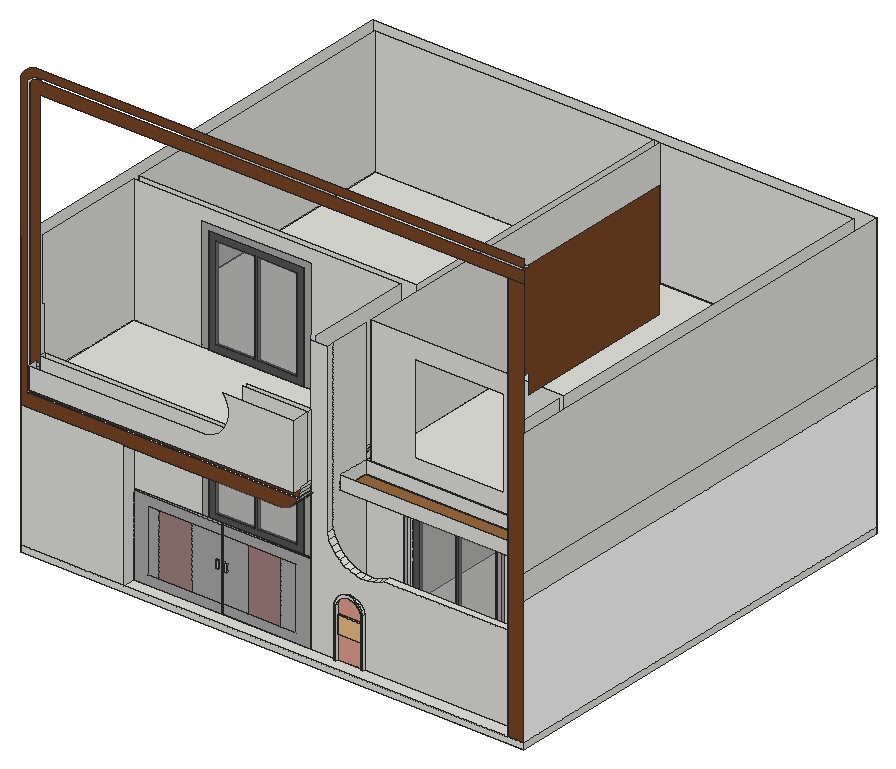
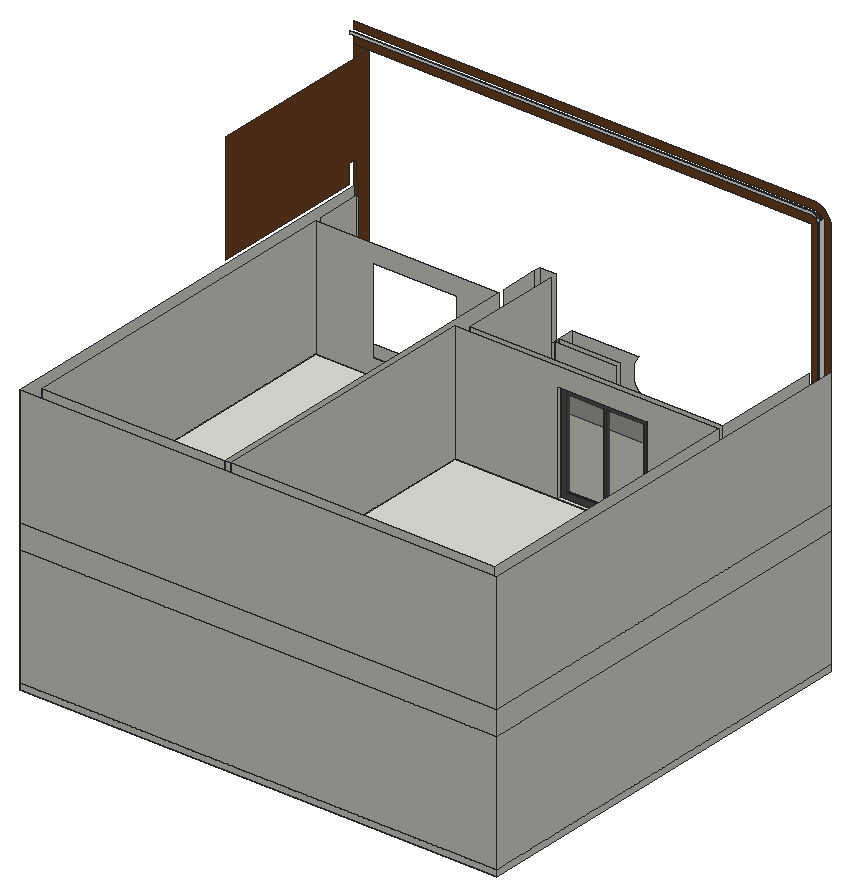
# SketchUp Ruby script. Lengths in millimetres.
U = 1.mm
M = Sketchup.active_model
def pt(a) = Geom::Point3d.new(a.map { |v| v * U })
def face(e, loops, mat)
  f = e.add_face(loops[0].map { |a| pt(a) })
  loops[1..].each { |l| e.add_face(l.map { |a| pt(a) }).erase! }
  f.material = f.back_material = mat if mat
  f
end
# faces: each face lists its corners as indices into pts; further lists are holes
def faces(e, pts, list, mat = nil) = list.each { |f| face(e, (f[0].is_a?(Array) ? f : [f]).map { |l| l.map { |i| pts[i] } }, mat) }
# xy, xz, yz: faces in a plane at the given z, y or x. An outline is a flat list of corners, or four numbers for a rectangle; further outlines are holes
def ring(l) = l.size == 4 ? [[l[0], l[1]], [l[2], l[1]], [l[2], l[3]], [l[0], l[3]]] : l.each_slice(2).to_a
def flat(e, list, mat, &to3) = list.each { |f| face(e, (f[0].is_a?(Array) ? f : [f]).map { |l| ring(l).map { |u, v| to3.(u, v) } }, mat) }
def xy(e, z, list, mat = nil) = flat(e, list, mat) { |x, y| [x, y, z] }
def xz(e, y, list, mat = nil) = flat(e, list, mat) { |x, z| [x, y, z] }
def yz(e, x, list, mat = nil) = flat(e, list, mat) { |y, z| [x, y, z] }
def lines(e, pts, list) = list.each { |a, b| e.add_line(pt(pts[a]), pt(pts[b])) }
# prism: a flat outline (further loops are holes) pulled along v
def prism(e, loops, v, mat = nil)
  f = face(e, loops, mat); d = Geom::Vector3d.new(v.map { |x| x * U })
  f.pushpull(f.normal.samedirection?(d) ? d.length : -d.length)
end
def box(e, o, s, mat = nil) = prism(e, [[o, [o[0] + s[0], o[1], o[2]], [o[0] + s[0], o[1] + s[1], o[2]], [o[0], o[1] + s[1], o[2]]]], [0, 0, s[2]], mat)
def at(x, y, z, deg = 0) = Geom::Transformation.translation(pt([x, y, z])) * Geom::Transformation.rotation(ORIGIN, Z_AXIS, deg.degrees)
def axes(o, x, y, z) = Geom::Transformation.new([*x, 0, *y, 0, *z, 0, *pt(o).to_a, 1])
def part(name) = M.definitions.add(name)
# library, detail: a bought-in or finely detailed component or shape, given as its bounding box
def library(name, o, s) = part(name).tap { |d| box(d.entities, o, s) }
def detail(e, o, s) = box(e.add_group.entities, o, s)
def put(e, d, t, mat = nil) = e.add_instance(d, t).tap { |i| i.material = mat if mat }
def group(e, t, mat = nil) = e.add_group.tap { |g| g.transformation = t; g.material = mat if mat }.entities
root = M.entities
M.materials.add("[0026_LightSalmon]").color = [225, 160, 143]
M.materials.add("[Color M00]").color = [255, 255, 255]
M.materials.add("[Color M03]").color = [170, 170, 170]
M.materials.add("[Color M06]").color = [86, 86, 86]
M.materials.add("[Metal Corrugated Shiny]").color = [193, 193, 193]
M.materials.add("[Translucent Glass Gray]").color = [128, 128, 128]
M.materials["[Translucent Glass Gray]"].alpha = 0.5
M.materials.add("[Wood Floor]").color = [155, 105, 61]
M.materials.add("[Wood Veneer 01]").color = [120, 70, 37]
M.materials.add("[Wood Veneer 02]").color = [163, 128, 128]
c1 = part("Group\#1")
xy(c1.entities,0,[[0,0,1355.7,60.3]],"[Color M06]")
xy(c1.entities,100.1,[[100.1,0,655.5,60.3],[696.9,0,1255.7,60.3]],"[Color M06]")
xy(c1.entities,1517.6,[[100.1,0,655.5,60.3],[696.9,0,1255.7,60.3]],"[Color M06]")
xy(c1.entities,1617.7,[[0,0,1355.7,60.3]],"[Color M06]")
xz(c1.entities,0,[[[0,0,1355.7,1617.7],[696.9,100.1,1255.7,1517.6],[100.1,100.1,655.5,1517.6]]],"[Color M06]")
xz(c1.entities,0,[[100.1,100.1,655.5,1517.6],[696.9,100.1,1255.7,1517.6]],"[Translucent Glass Gray]")
xz(c1.entities,60.3,[[[0,0,1355.7,1617.7],[696.9,100.1,1255.7,1517.6],[100.1,100.1,655.5,1517.6]]],"[Color M06]")
yz(c1.entities,0,[[0,0,60.3,1617.7]],"[Color M06]")
yz(c1.entities,100.1,[[0,100.1,60.3,1517.6]],"[Color M06]")
yz(c1.entities,655.5,[[0,100.1,60.3,1517.6]],"[Color M06]")
yz(c1.entities,696.9,[[0,100.1,60.3,1517.6]],"[Color M06]")
yz(c1.entities,1255.7,[[0,100.1,60.3,1517.6]],"[Color M06]")
yz(c1.entities,1355.7,[[0,0,60.3,1617.7]],"[Color M06]")
c2 = library("61A",[37.8,0,0],[1466.5,605.7,101.6])
xy(root,0,[[3.3,209.6,12195.3,10877.6]])
xy(root,152.4,[[[3.3,209.6,3.3,10877.6,12195.3,10877.6,12195.3,209.6,11814.3,209.6,11814.3,514.4,11890.5,514.4,11890.5,687.4,6787.6,687.4,6787.6,3257.6,4426,3257.6,4426,3410,7047,3410,7047,10572.8,7199.4,10572.8,7199.4,1809.8,11890.5,1809.8,11890.5,10572.8,308.1,10572.8,308.1,3410,2137.7,3410,2137.7,3257.6,308.1,3257.6,308.1,514.4,2505.2,514.4,2505.2,209.6],[7199.4,698.5,11890.5,1657.4]],[2505.2,209.6,11814.3,209.6,11814.3,514.4,8100.8,514.4,8100.8,463.6,8038.4,463.6,8038.4,514.4,7446.1,514.4,7446.1,463.6,7383.6,463.6,7383.6,514.4,2505.2,514.4],[7383.6,463.6,7446.1,514.4],[8038.4,463.6,8100.8,514.4],[308.1,514.4,6787.6,3257.6],
  [6787.6,514.4,11890.5,687.4],[7199.4,698.5,11890.5,1657.4],[7199.4,1809.8,11890.5,10572.8],[2137.7,3257.6,4426,3410],[308.1,3410,7047,10572.8]])
xy(root,543.9,[[8185.1,1603.4,10552.1,1657.4]])
xy(root,759.3,[[8275.8,1657.4,10434.8,1809.8]])
xy(root,759.3,[[8275.8,1603.4,10434.8,1657.4]],"[Color M03]")
xy(root,2234.1,[[8561.3,514.4,11890.5,687.4]])
xy(root,2700.1,[[2137.7,3257.5,4426,3409.9]])
xy(root,3162.7,[[8275.8,1603.4,10434.8,1657.4],[8275.8,1657.4,10434.8,1809.8]])
xy(root,3200.4,[[2505.2,209.6,2505.2,514.4,308.1,514.4,308.1,3257.6,6237.2,3257.6,6237.2,209.6]])
xy(root,3271.3,[[8185.1,1603.4,10552.1,1657.4]],"[Color M03]")
xy(root,3514.6,[[181.8,209.6,6734,325.4]],"[Color M00]")
xy(root,3559,[[241.3,209.6,6734,325.4]],"[Color M00]")
xy(root,3584.1,[[7199.4,887.4,11890.5,1657.4]],"[Wood Floor]")
xy(root,3752.8,[[374.7,0,6787.6,209.6]])
xy(root,3810,[[308.1,424.6,6787.6,555.6],[308.1,555.6,6787.6,555.6,6787.6,3257.6,4426,3257.6,2137.7,3257.5,1971.4,3257.5,308.1,3257.6],[7199.4,1809.8,11890.5,10572.8],[2137.7,3257.5,4426,3257.6,4426,3410,2137.7,3410],[308.1,3410,7047,10572.8]])
xz(root,0,[[374.7,3752.8,6787.6,3752.8,6787.6,5334,5080.9,5334,5145.9,5230.5,5190.6,5116.7,5213.7,4996.7,5214.2,4874.4,5192.2,4754.2,5148.4,4640.1,5084.4,4536,5002.2,4445.4,4904.8,4371.6,4795.5,4317,4677.9,4283.4,4556.2,4272.1,374.7,4272.1]])
xz(root,209.6,[[3.3,0,12195.3,152.4],[3.3,152.4,2505.2,3200.4],[374.7,3752.8,6787.6,3810]])
xz(root,209.6,[[11814.3,152.4,12195.3,10096.5],[3.3,3200.4,6237.2,3200.4,6314.1,3205.8,6389.5,3221.8,6461.9,3248.1,6530,3284.2,6592.3,3329.4,6647.8,3382.9,6695.4,3443.6,6734,3510.2,6763,3581.6,6781.8,3656.4,6790,3733,6787.6,3810,6787.6,3752.8,374.7,3752.8,374.7,4272.1,479.5,4272.1,479.5,10096.5,12195.3,10096.5,12195.3,10388.1,531,10388.1,503.8,10394.3,476.2,10397.6,448.3,10397.9,420.5,10395,393.2,10389.2,366.8,10380.4,341.4,10368.8,317.5,10354.5,295.2,10337.7,275,10318.5,257,10297.2,241.3,10274.1,241.3,3559,6734,3559,6734,3514.6,181.8,3514.6,181.8,10303.9,202.4,10329.9,219.1,10347.4,225.2,10353.9,250.2,10375.7,277.2,10395,305.8,10411.7,335.8,10425.7,367.1,10436.8,399.2,10444.9,431.9,10450,465,10452,498.1,10450.9,531,10446.7,12195.3,10446.7,12195.3,10642.6,432,10642.6,373.3,10634.9,306.3,10615.8,242.9,10587,184.5,10549,132.4,10502.9,87.7,10449.5,51.4,10390.1,24.3,10325.9,7.1,10258.4,3.3,10221.2]],"[Wood Veneer 01]")
xz(root,325.4,[[181.8,3514.6,6734,3514.6,6734,3559,241.3,3559,241.3,10274.1,257,10297.2,275,10318.5,295.2,10337.7,317.5,10354.5,341.4,10368.8,366.8,10380.4,393.2,10389.2,420.5,10395,448.3,10397.9,476.2,10397.6,503.8,10394.3,531,10388.1,12195.3,10388.1,12195.3,10446.7,531,10446.7,498.1,10450.9,465,10452,431.9,10450,399.2,10444.9,367.1,10436.8,335.8,10425.7,305.8,10411.7,277.2,10395,250.2,10375.7,225.2,10353.9,219.1,10347.4,202.4,10329.9,181.8,10303.9]],"[Color M00]")
xz(root,424.6,[[308.1,3810,6787.6,3810,6787.6,5334,5214.2,5334,5214.2,4272.1,308.1,4272.1]])
xz(root,463.6,[[7383.6,152.4,7446.1,152.4,7446.1,1349.5,7467.8,1414.6,7503.5,1473.1,7551.6,1522,7609.4,1558.9,7674.1,1581.8,7742.2,1589.6,7810.4,1581.8,7875,1558.9,7932.8,1522,7980.9,1473.1,8016.7,1414.6,8038.4,1349.5,8038.4,152.4,8100.8,152.4,8100.8,1359.7,8073.6,1441.1,8030.4,1511.7,7972.4,1570.8,7902.6,1615.4,7824.5,1643,7742.2,1652.4,7659.9,1643,7581.9,1615.4,7512,1570.8,7454,1511.7,7410.8,1441.1,7383.6,1359.7]])
xz(root,514.4,[[7383.6,90,8100.8,152.4],[308.1,152.4,2505.2,3200.4],[6787.6,152.4,7383.6,152.4,7383.6,1359.7,7410.8,1441.1,7454,1511.7,7512,1570.8,7581.9,1615.4,7659.9,1643,7742.2,1652.4,7824.5,1643,7902.6,1615.4,7972.4,1570.8,8030.4,1511.7,8073.6,1441.1,8100.8,1359.7,8100.8,152.4,11814.3,152.4,11814.3,2234.1,8561.3,2234.1,8432.1,2170,8294.4,2127,8151.7,2106.2,8007.5,2108.2,7865.3,2132.9,7728.9,2179.6,7601.5,2247.2,7486.3,2334.1,7386.2,2438,7303.8,2556.3,7241,2686.2,7199.4,2824.3,7199.4,6858,6787.6,6858,6787.6,3810,6790,3733,6787.6,3709.8],[7383.6,152.4,7383.6,1359.7,7410.8,1441.1,7454,1511.7,7512,1570.8,7581.9,1615.4,7659.9,1643,7742.2,1652.4,7824.5,1643,7902.6,1615.4,7972.4,1570.8,8030.4,1511.7,8073.6,1441.1,8100.8,1359.7,8100.8,152.4,8038.4,152.4,8038.4,1349.5,8016.7,1414.6,7980.9,1473.1,7932.8,1522,7875,1558.9,7810.4,1581.8,7742.2,1589.6,7674.1,1581.8,7609.4,1558.9,7551.6,1522,7503.5,1473.1,7467.8,1414.6,7446.1,1349.5,7446.1,152.4],[11814.3,152.4,11890.5,2234.1],
  [11814.3,2234.1,11890.5,2824.3],[11814.3,2824.3,11890.5,6858]])
xz(root,514.4,[[7446.1,152.4,8038.4,152.4,8038.4,1349.5,8016.7,1414.6,7980.9,1473.1,7932.8,1522,7875,1558.9,7810.4,1581.8,7742.2,1589.6,7674.1,1581.8,7609.4,1558.9,7551.6,1522,7503.5,1473.1,7467.8,1414.6,7446.1,1349.5]],"[0026_LightSalmon]")
xz(root,555.6,[[308.1,3810,308.1,4272.1,5214.2,4272.1,5214.2,5334,6787.6,5334,6787.6,3810]])
xz(root,887.4,[[7199.4,3584.1,11890.5,3899.4]])
xz(root,1603.4,[[[8185.1,543.9,10552.1,3271.3],[8275.8,759.3,10434.8,3162.7]]],"[Color M03]")
xz(root,1657.4,[[[7199.4,152.4,11890.5,3584.1],[8185.1,543.9,10552.1,3271.3]],[[8185.1,543.9,10552.1,3271.3],[8275.8,759.3,10434.8,3162.7]],[7199.4,3584.1,11890.5,3899.4]])
xz(root,1809.8,[[[7199.4,152.4,11890.5,3200.4],[8275.8,759.3,10434.8,3162.7]],[7199.4,3200.4,11890.5,3810]])
xz(root,3257.6,[[6787.6,3709.8,6787.6,3810,6790,3733]])
xz(root,3410,[[308.1,3200.4,7047,3810],[308.1,3810,308.1,6858,7047,6858,7047,3810,4426,3810,4426,6383.1,2137.7,6383.1,2137.7,3810]])
xz(root,10572.8,[[308.1,152.4,7047,3200.4],[7047,152.4,7199.4,3200.4],[7199.4,152.4,11890.5,3200.4],[308.1,3200.4,7047,3810],[7047,3200.4,7199.4,3810],
  [7199.4,3200.4,11890.5,3810],[308.1,3810,7047,6858],[7047,3810,7199.4,6858],[7199.4,3810,11890.5,6858]])
xz(root,10877.6,[[3.3,0,12195.3,152.4],[3.3,152.4,12195.3,3200.4],[3.3,3200.4,12195.3,3810],[3.3,3810,12195.3,6858]])
yz(root,3.3,[[209.6,0,10877.6,152.4],[209.6,152.4,10877.6,3200.4],[209.6,3200.4,10877.6,3810],[209.6,3810,10877.6,6858]])
yz(root,181.8,[[209.6,3514.6,325.4,10303.9]],"[Color M00]")
yz(root,241.3,[[209.6,3559,325.4,10274.1]],"[Color M00]")
yz(root,308.1,[[514.4,152.4,3257.6,3200.4],[3410,152.4,10572.8,3200.4],[514.4,3200.4,3257.6,3810],[3410,3200.4,10572.8,3810],[424.6,3810,555.6,4272.1],
  [555.6,3810,3257.6,3810,3257.6,6858,514.4,6858,514.4,5372.1,555.6,5372.1],[3410,3810,10572.8,6858]])
yz(root,374.7,[[0,3752.8,209.6,4272.1]])
yz(root,2137.7,[[3257.6,152.4,3410,152.4,3409.9,2700.1,3257.5,2700.1],[3257.5,3810,3410,6383.1]])
yz(root,2505.2,[[209.6,152.4,514.4,3200.4]])
yz(root,4426,[[3257.6,152.4,3257.5,2700.1,3409.9,2700.1,3410,152.4],[3257.6,3810,3257.5,6383.1,3410,6383.1,3410,3810]])
yz(root,6734,[[209.6,3514.6,325.4,3559]],"[Color M00]")
yz(root,6787.6,[[514.4,152.4,687.4,3709.8],[687.4,152.4,3257.6,3709.8],[0,3752.8,209.6,3752.8,209.6,3810,424.6,3810,424.6,5334,0,5334],[424.6,3810,514.4,5334],[514.4,3810,555.6,5334],
  [555.6,3810,687.4,5334],[687.4,3810,3257.6,6858]])
yz(root,7047,[[3410,152.4,10572.8,3200.4],[3410,3200.4,10572.8,3810],[3410,3810,10572.8,6858]])
yz(root,7199.4,[[698.5,152.4,1657.4,152.4,1657.4,3584.1,887.4,3584.1,887.4,3899.4,1657.4,3899.4,1657.4,6858,687.4,6858,687.4,2824.3,698.5,2824.3],[1809.8,152.4,10572.8,3200.4],[514.4,2824.3,687.4,6858],[1809.8,3200.4,10572.8,3810],[887.4,3584.1,1657.4,3899.4],
  [1809.8,3810,10572.8,6858]])
yz(root,7383.6,[[463.6,152.4,514.4,1359.7]])
yz(root,7446.1,[[463.6,152.4,514.4,1349.5]])
yz(root,8038.4,[[463.6,152.4,514.4,1349.5]])
yz(root,8100.8,[[463.6,152.4,514.4,1359.7]])
yz(root,8185.1,[[1603.4,543.9,1657.4,3271.3]],"[Color M03]")
yz(root,8275.8,[[1603.4,759.3,1657.4,3162.7],[1657.4,759.3,1809.8,3162.7]])
yz(root,10434.8,[[1657.4,759.3,1809.8,3162.7]])
yz(root,10434.8,[[1603.4,759.3,1657.4,3162.7]],"[Color M03]")
yz(root,10552.1,[[1603.4,543.9,1657.4,3271.3]],"[Color M03]")
yz(root,11814.3,[[209.6,152.4,209.6,10096.5,4760.9,10096.5,4760.9,7289.8,849.3,7289.8,849.3,7765.4,642.9,7765.4,642.9,8839.2,606.3,8839.2,606.3,7765.4,582.5,7765.4,582.5,7289.8,514.4,7289.8,514.4,152.4]],"[Wood Veneer 01]")
yz(root,11890.5,[[514.4,152.4,687.4,2234.1],[698.5,152.4,698.5,2824.3,514.4,2824.3,514.4,6858,1657.4,6858,1657.4,3899.4,1049.4,3899.4,1049.4,5423.4,946.6,5423.4,946.6,3899.4,887.4,3899.4,887.4,3584.1,1657.4,3584.1,1657.4,152.4],[1809.8,152.4,10572.8,3200.4],[1809.8,3200.4,10572.8,3810],[887.4,3584.1,1657.4,3899.4],
  [1809.8,3810,10572.8,6858]])
yz(root,12195.3,[[209.6,0,10877.6,152.4],[209.6,3200.4,10877.6,3810],[209.6,3810,10877.6,6858]])
yz(root,12195.3,[[209.6,152.4,10877.6,3200.4]],"[Color M00]")
p = [[1988.4,3257.6,152.4],[1988.4,3257.6,3.1],[4575.2,3257.6,3.1],[4575.2,3257.6,152.4],[4426,3257.6,152.4],[4426,3257.6,127],
  [2137.7,3257.5,127],[2137.7,3257.6,152.4],[308.1,3257.6,152.4],[1988.4,3257.5,2849.3],[4575.2,3257.5,2849.3],[6787.6,3257.6,152.4],
  [6787.6,3257.6,3709.8],[6781.8,3257.6,3656.4],[6763,3257.6,3581.6],[6734,3257.6,3510.2],[6695.4,3257.6,3443.6],[6647.8,3257.6,3382.9],
  [6592.3,3257.6,3329.4],[6530,3257.6,3284.2],[6461.9,3257.6,3248.1],[6389.5,3257.6,3221.8],[6314.1,3257.6,3205.8],[6237.2,3257.6,3200.4],
  [308.1,3257.6,3200.4],[2137.7,3257.5,2700.1],[4426,3257.5,2700.1],[7047,3410,152.4],[4426,3410,152.4],[4426,3409.9,2700.1],
  [2137.7,3409.9,2700.1],[2137.7,3410,152.4],[308.1,3410,152.4],[308.1,3410,3200.4],[7047,3410,3200.4],[7446.1,514.4,1349.5],
  [7467.8,514.4,1414.6],[7467.8,463.6,1414.6],[7446.1,463.6,1349.5],[8016.7,514.4,1414.6],[8038.4,514.4,1349.5],[8038.4,463.6,1349.5],
  [8016.7,463.6,1414.6],[7410.8,514.4,1441.1],[7383.6,514.4,1359.7],[7383.6,463.6,1359.7],[7410.8,463.6,1441.1],[8100.8,514.4,1359.7],
  [8073.6,514.4,1441.1],[8073.6,463.6,1441.1],[8100.8,463.6,1359.7],[7503.5,514.4,1473.1],[7503.5,463.6,1473.1],[7980.9,514.4,1473.1],
  [7980.9,463.6,1473.1],[7454,514.4,1511.7],[7454,463.6,1511.7],[8030.4,514.4,1511.7],[8030.4,463.6,1511.7],[7551.6,514.4,1522],
  [7551.6,463.6,1522],[7932.8,514.4,1522],[7932.8,463.6,1522],[7512,514.4,1570.8],[7512,463.6,1570.8],[7972.4,514.4,1570.8],
  [7972.4,463.6,1570.8],[7609.4,514.4,1558.9],[7609.4,463.6,1558.9],[7875,514.4,1558.9],[7875,463.6,1558.9],[7674.1,514.4,1581.8],
  [7674.1,463.6,1581.8],[7810.4,514.4,1581.8],[7810.4,463.6,1581.8],[7581.9,514.4,1615.4],[7581.9,463.6,1615.4],[7902.6,514.4,1615.4],
  [7902.6,463.6,1615.4],[7742.2,514.4,1589.6],[7742.2,463.6,1589.6],[7659.9,514.4,1643],[7659.9,463.6,1643],[7824.5,514.4,1643],
  [7824.5,463.6,1643],[7742.2,514.4,1652.4],[7742.2,463.6,1652.4],[8007.5,514.4,2108.2],[8151.7,514.4,2106.2],[8151.7,687.4,2106.2],
  [8007.5,687.4,2108.2],[8294.4,514.4,2127],[8294.4,687.4,2127],[7865.3,514.4,2132.9],[7865.3,687.4,2132.9],[8432.1,514.4,2170],
  [8432.1,687.4,2170],[7728.9,514.4,2179.6],[7728.9,687.4,2179.6],[8561.3,514.4,2234.1],[8561.3,687.4,2234.1],[7601.5,514.4,2247.2],
  [7601.5,687.4,2247.2],[7486.3,514.4,2334.1],[7486.3,687.4,2334.1],[7386.2,514.4,2438],[7386.2,687.4,2438],[7303.8,514.4,2556.3],
  [7303.8,687.4,2556.3],[7241,514.4,2686.2],[7241,687.4,2686.2],[7199.4,514.4,2824.3],[7199.4,687.4,2824.3],[6314.1,209.6,3205.8],
  [6237.2,209.6,3200.4],[308.1,3257.6,3810],[1971.4,3257.5,3810],[1971.4,3257.5,3643.7],[4592.3,3257.5,3643.7],[4592.3,3257.6,3810],
  [6787.6,3257.6,3810],[6389.5,209.6,3221.8],[6461.9,209.6,3248.1],[6530,209.6,3284.2],[6592.3,209.6,3329.4],[6647.8,209.6,3382.9],
  [6695.4,209.6,3443.6],[6734,209.6,3510.2],[6763,209.6,3581.6],[6781.8,209.6,3656.4],[4426,3257.6,3810],[2137.7,3257.5,3810],
  [6787.6,687.4,3709.8],[6787.6,514.4,3709.8],[6790,514.4,3733],[6790,209.6,3733],[6790,687.4,3733],[6790,3257.6,3733],
  [6787.6,514.4,3810],[6787.6,424.6,3810],[6787.6,209.6,3810],[6787.6,687.4,3810],[6787.6,555.6,3810],[11890.5,1809.8,3810],
  [7199.4,1809.8,3810],[7199.4,1809.8,6858],[11890.5,1809.8,6858],[8275.8,1809.7,4242.9],[10434.8,1809.7,4242.9],[10434.8,1809.7,6401.9],
  [8275.8,1809.7,6401.9],[1971.4,3257.5,6549.4],[4592.3,3257.5,6549.4],[6787.6,3257.6,6858],[308.1,3257.6,6858],[2137.7,3257.5,6383.1],
  [4426,3257.5,6383.1],[308.1,209.6,3810],[308.1,424.6,3810]]
faces(root,p,[[0,1,2,3,4,5,6,7],[5,4,7,6],[8,0,9,10,3,11,12,13,14,15,16,17,18,19,20,21,22,23,24],[27,28,29,30,31,32,33,34],[35,36,37,38],[39,40,41,42],[43,44,45,46],[47,48,49,50],
  [36,51,52,37],[53,39,42,54],[55,43,46,56],[48,57,58,49],[51,59,60,52],[61,53,54,62],[63,55,56,64],[57,65,66,58],
  [59,67,68,60],[69,61,62,70],[67,71,72,68],[73,69,70,74],[75,63,64,76],[65,77,78,66],[71,79,80,72],[79,73,74,80],
  [81,75,76,82],[77,83,84,78],[85,81,82,86],[83,85,86,84],[87,88,89,90],[88,91,92,89],[93,87,90,94],[91,95,96,92],
  [97,93,94,98],[95,99,100,96],[101,97,98,102],[103,101,102,104],[105,103,104,106],[107,105,106,108],[109,107,108,110],[111,109,110,112],
  [23,22,113,114],[115,116,117,118,119,120,12,13,14,15,16,17,18,19,20,21,22,23,24],[22,21,121,113],[21,20,122,121],[20,19,123,122],[19,18,124,123],[18,17,125,124],[17,16,126,125],
  [16,15,127,126],[15,14,128,127],[14,13,129,128],[130,119,118,117,116,131],[13,12,132,133,134,135,129],[134,133,132,136],[12,137,136,132],[135,134,138,139,140],
  [138,134,136,141,142],[137,120,141,136],[[143,144,145,146],[147,148,149,150]],[115,116,151,152,119,120,153,154]])
faces(root,p,[[4,3,10,9,0,7,25,26],[130,119,152,151,116,131,155,156]],"[Color M03]")
lines(root,p,[[157,158]])
put(root,c1,axes([2137.7,3257.5,152.4],[1.68788,0,0],[0,0.84,0],[0,0,1.59062]))
g1 = group(root,at(2505.2,489,152.4))
xy(g1,0,[[0,25.4,0,96.8,4282.4,96.8,4282.4,25.4,2148.4,25.4,2148.4,33.3,2127.2,33.3,2127.2,25.4]],"[Color M03]")
xy(g1,958.5,[[2004.6,0,2069.7,23.8],[2204.8,0,2269.9,23.8]],"[Color M03]")
xy(g1,971.9,[[2004.6,15.9,2069.7,23.8]],"[Color M03]")
xy(g1,994.3,[[2204.8,15.9,2269.9,23.8]],"[Color M03]")
xy(g1,1106.1,[[2004.6,15.9,2069.7,25.4],[2204.8,15.9,2269.9,25.4]],"[Color M03]")
xy(g1,1147.4,[[2004.6,0,2069.7,25.4],[2204.8,0,2269.9,25.4]],"[Metal Corrugated Shiny]")
xy(g1,1941.5,[[0,25.4,2127.2,25.4,2127.2,33.3,2148.4,33.3,2148.4,25.4,4282.4,25.4,4282.4,96.8,0,96.8]],"[Color M03]")
xz(g1,0,[[2004.6,958.5,2069.7,1147.4],[2204.8,958.5,2269.9,1147.4]],"[Metal Corrugated Shiny]")
xz(g1,15.9,[[2004.6,971.9,2069.7,1106.1],[2204.8,994.3,2269.9,1106.1]],"[Color M03]")
xz(g1,23.8,[[2004.6,958.5,2069.7,971.9],[2204.8,958.5,2269.9,994.3]],"[Color M03]")
xz(g1,25.4,[[0,0,2127.2,0,2127.2,223,351.5,223,351.5,1718.5,2127.2,1718.5,2127.2,1941.5,0,1941.5],[2148.4,0,4282.4,0,4282.4,1941.5,2148.4,1941.5,2148.4,1718.5,3930.9,1718.5,3930.9,223,2148.4,223],[351.5,223,603.4,1718.5],[[1402.3,223,2127.2,1718.5],[2004.6,1106.1,2069.7,1147.4]],[[2148.4,223,2758.4,1718.5],[2204.8,1106.1,2269.9,1147.4]],
  [3557.2,223,3930.9,1718.5],[2004.6,1106.1,2069.7,1147.4],[2204.8,1106.1,2269.9,1147.4]],"[Color M03]")
xz(g1,25.4,[[603.4,223,1402.3,1718.5],[2758.4,223,3557.2,1718.5]],"[Wood Veneer 02]")
xz(g1,33.3,[[2127.2,0,2148.4,1941.5]],"[Color M03]")
xz(g1,96.8,[[0,0,4282.4,1941.5]],"[Color M03]")
yz(g1,0,[[25.4,0,96.8,1941.5]],"[Color M03]")
yz(g1,2004.6,[[0,958.5,0,1147.4,25.4,1147.4,25.4,1106.1,15.9,1106.1,15.9,971.9,23.8,971.9,23.8,958.5]],"[Metal Corrugated Shiny]")
yz(g1,2069.7,[[0,958.5,23.8,958.5,23.8,971.9,15.9,971.9,15.9,1106.1,25.4,1106.1,25.4,1147.4,0,1147.4]],"[Metal Corrugated Shiny]")
yz(g1,2127.2,[[25.4,0,33.3,223],[25.4,223,33.3,1718.5],[25.4,1718.5,33.3,1941.5]],"[Color M03]")
yz(g1,2148.4,[[25.4,0,33.3,223],[25.4,223,33.3,1718.5],[25.4,1718.5,33.3,1941.5]],"[Color M03]")
yz(g1,2204.8,[[0,958.5,0,1147.4,25.4,1147.4,25.4,1106.1,15.9,1106.1,15.9,994.3,23.8,994.3,23.8,958.5]],"[Metal Corrugated Shiny]")
yz(g1,2269.9,[[0,958.5,23.8,958.5,23.8,994.3,15.9,994.3,15.9,1106.1,25.4,1106.1,25.4,1147.4,0,1147.4]],"[Metal Corrugated Shiny]")
yz(g1,4282.4,[[25.4,0,96.8,1941.5]],"[Color M03]")
p = [[2148.4,33.3,1718.5],[2148.4,96.8,1718.5],[2148.4,33.3,223],[2148.4,96.8,223],[2127.2,33.3,223],[2127.2,96.8,223],
  [603.4,25.4,1718.5],[603.4,96.8,1718.5],[603.4,25.4,223],[603.4,96.8,223],[351.5,25.4,1718.5],[351.5,96.8,1718.5],
  [3930.9,25.4,223],[3930.9,96.8,223],[3930.9,25.4,1718.5],[3930.9,96.8,1718.5],[2758.4,25.4,223],[2758.4,96.8,223],
  [3557.2,25.4,1718.5],[3557.2,96.8,1718.5],[3557.2,25.4,223],[3557.2,96.8,223],[2758.4,25.4,1718.5],[2758.4,96.8,1718.5],
  [1402.3,25.4,1718.5],[1402.3,96.8,1718.5],[1402.3,25.4,223],[1402.3,96.8,223]]
lines(g1,p,[[0,1],[2,3],[4,5],[6,7],[8,9],[10,11],[12,13],[14,15],[16,17],[18,19],[20,21],[22,23],
  [24,25],[26,27]])
put(root,c2,axes([7476.9,463.5,745.3],[0.37,0,0],[0,0,0.69],[0,0.5,0]))
put(root,c1,axes([8275.8,1749.4,759.3],[1.59251,0,0],[0,1,0],[0,0,1.48577]))
put(root,c1,axes([2137.7,3257.5,3810],[1.68788,0,0],[0,0.84,0],[0,0,1.59062]))
